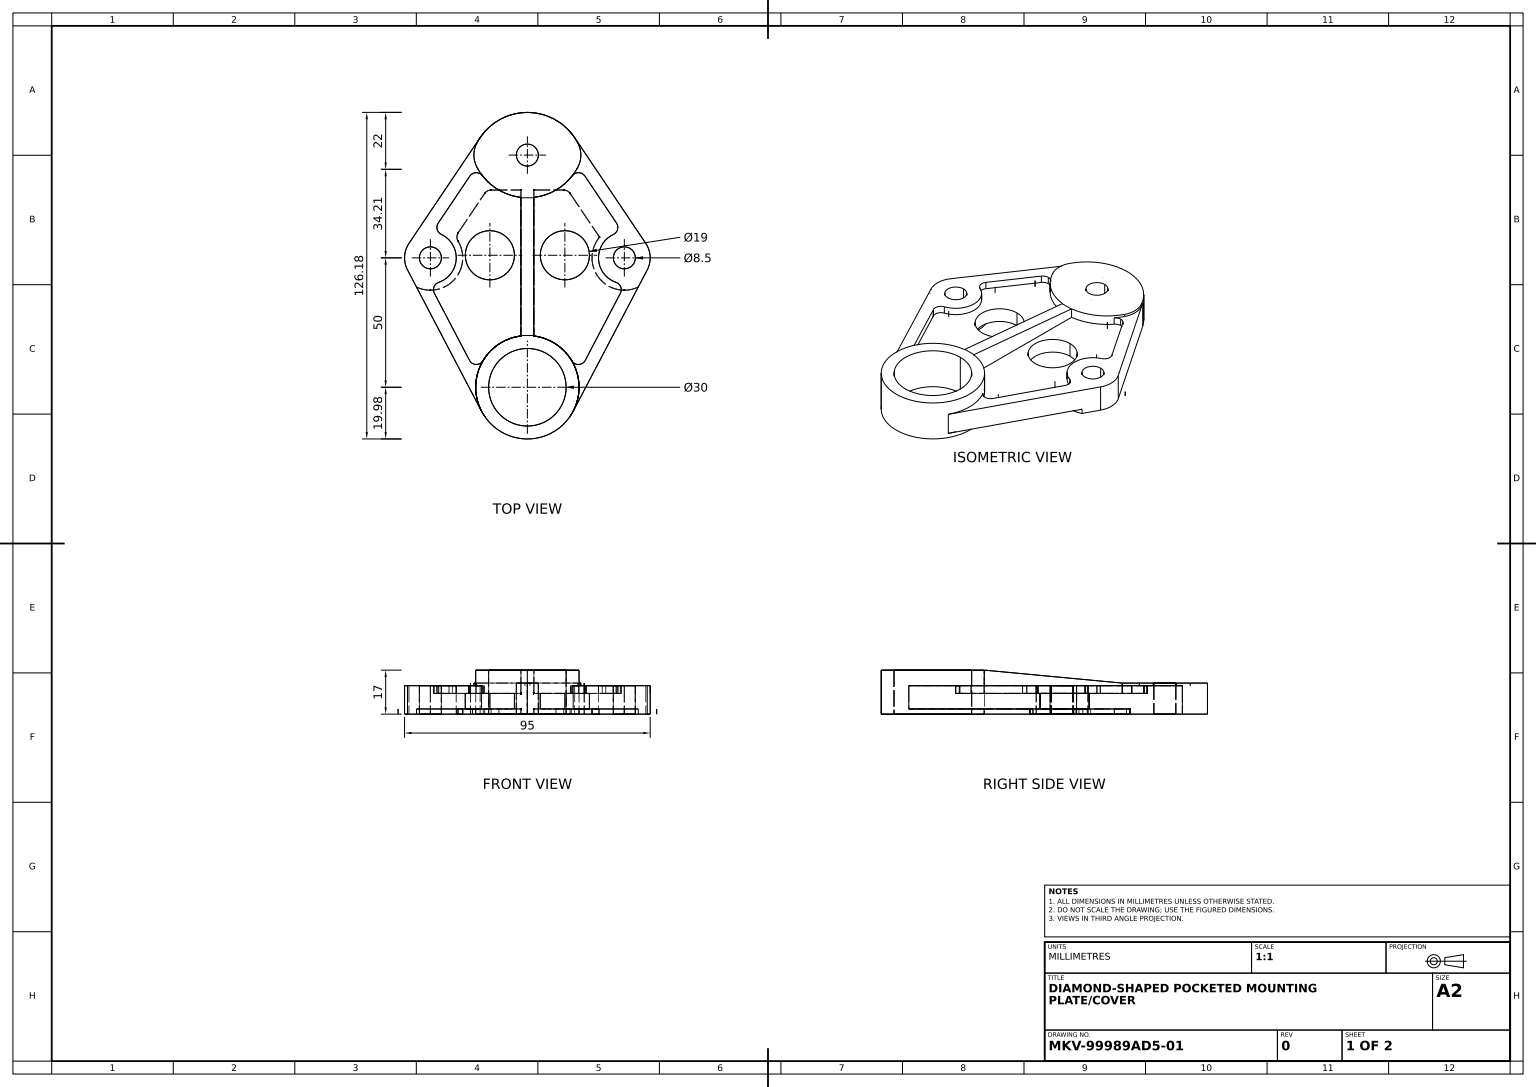
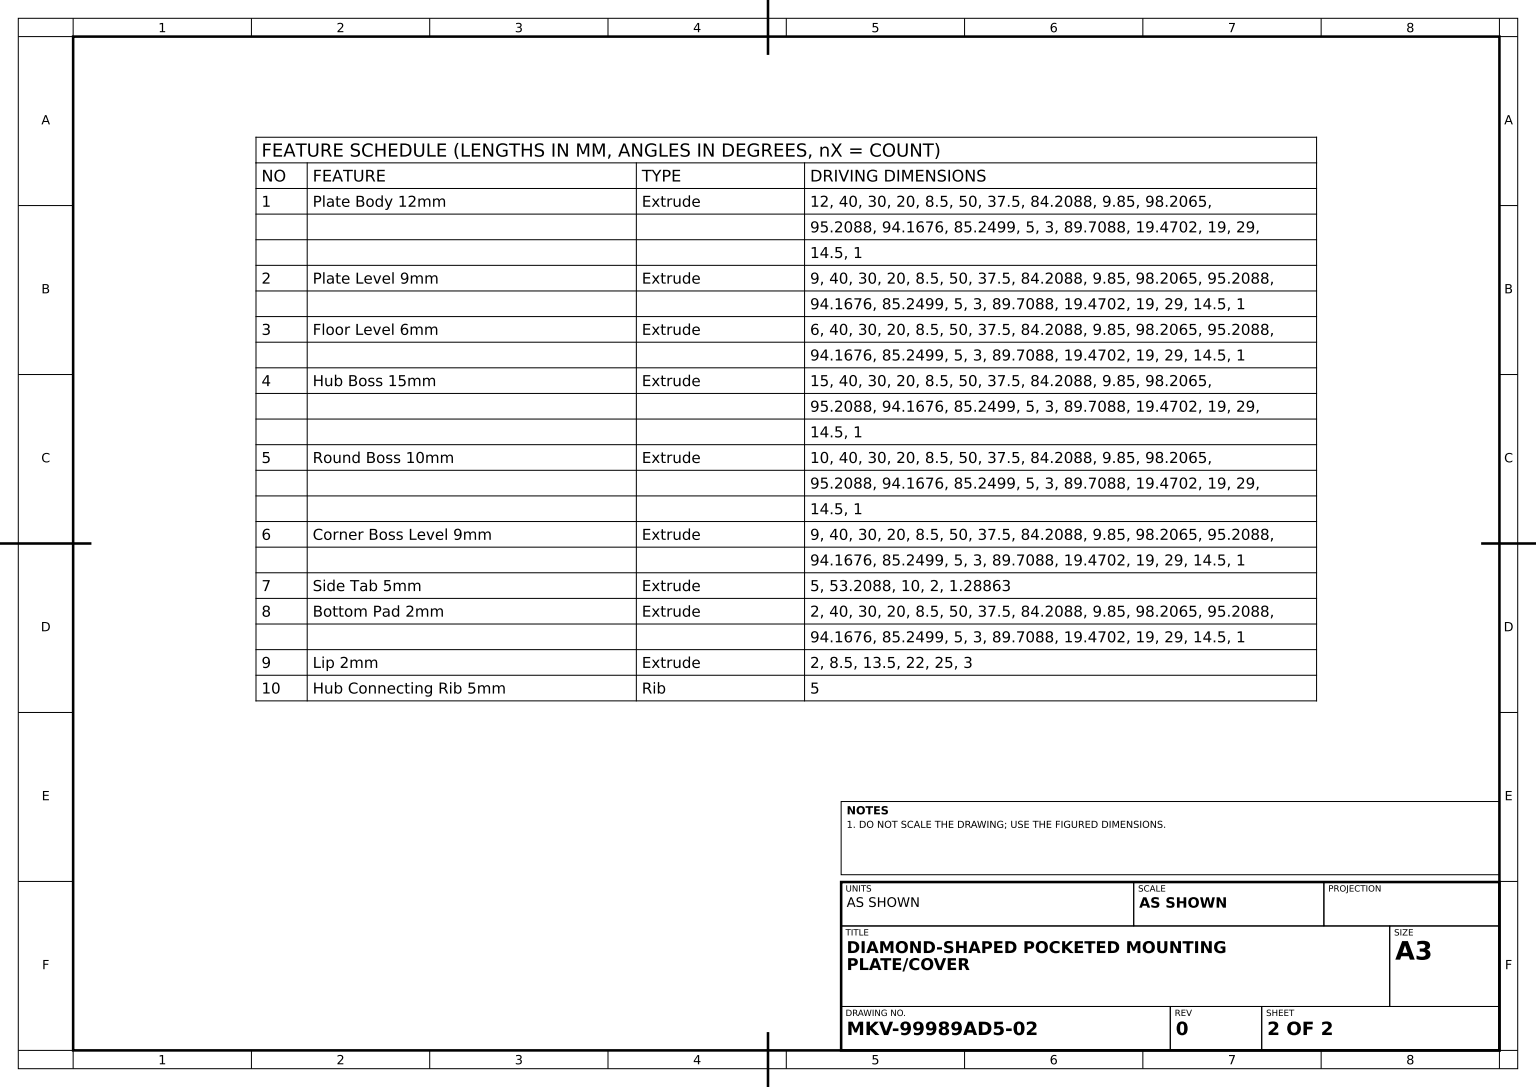
solid
v1 (-26.813948518,0,-56.485237369)
v2 (-37.5,0,-37.5)
e1 v1 v2 CIRCLE(AX(P(-37.5,0,-50),D(0,-1,0),D(0,0,-1)),12.5)
v3 (-37.5,-2,-37.5)
e2 v3 v2 LINE
v4 (-26.813948518,-2,-56.485237369)
e3 v4 v3 CIRCLE(AX(P(-37.5,-2,-50),D(0,-1,0),D(0,0,-1)),12.5)
e4 v4 v1 LINE
face CYL(AX(P(-37.5,-2,-50),D(0,1,0),D(0,0,1)),12.5) [e1 -e2 -e3 e4]
v5 (2.5,0,-19.843134833)
v6 (2.5,-2,-19.843134833)
e5 v5 v6 LINE
v7 (2.5,-2,-76.208782064)
e6 v7 v6 LINE
v8 (2.5,0,-76.208782064)
e7 v7 v8 LINE
e8 v8 v5 LINE
face PLANE(AX(P(2.5,-2,-20),D(-1,0,0),D(0,0,1))) rev [e5 -e6 e7 e8]
v9 (-14.5,0,-60.5)
v10 (-14.5,0,-41.5)
e9 v9 v10 CIRCLE(AX(P(-14.5,0,-51),D(0,1,0),D(0,0,1)),9.5)
e10 v10 v9 CIRCLE(AX(P(-14.5,0,-51),D(0,1,0),D(0,0,1)),9.5)
v11 (-26.737782046,0,-59.717235446)
e11 v1 v11 CIRCLE(AX(P(-24.249296162,0,-58.041694337),D(0,-1,0),D(0,0,-1)),3)
v12 (-16.525516364,0,-74.884323173)
e12 v11 v12 LINE
v13 (-14.037030481,0,-76.208782064)
e13 v13 v12 CIRCLE(AX(P(-14.037030481,0,-73.208782064),D(0,1,0),D(0,0,-1)),3)
v14 (-2.5,0,-76.208782064)
e14 v13 v14 LINE
v15 (-2.5,0,-19.843134833)
e15 v14 v15 LINE
v16 (-17.713872229,0,9.285404172)
e16 v15 v16 CIRCLE(AX(P(0,0,0),D(0,1,0),D(0,0,1)),20)
v17 (-42.87490955,0,-38.714595828)
e17 v17 v16 LINE
e18 v2 v17 CIRCLE(AX(P(-37.5,0,-50),D(0,-1,0),D(0,0,-1)),12.5)
face PLANE(AX(P(0,0,0),D(0,1,0),D(0,0,1))) rev [e9 e10] [-e1 e11 e12 -e13 e14 e15 e16 -e17 -e18]
v18 (-45.794952945,9,-55.58513703)
v19 (-46.356936115,9,-45.357297914)
e19 v18 v19 CIRCLE(AX(P(-37.5,9,-50),D(0,1,0),D(0,0,1)),10)
v20 (-45.794952945,-2,-55.58513703)
e20 v18 v20 LINE
v21 (-46.356936115,-2,-45.357297914)
e21 v21 v20 CIRCLE(AX(P(-37.5,-2,-50),D(0,-1,0),D(0,0,-1)),10)
e22 v19 v21 LINE
face CYL(AX(P(-37.5,6,-50),D(0,-1,0),D(0,0,-1)),10) [-e19 e20 -e21 -e22]
v22 (19.772275057,6,-82.909855988)
v23 (17.39960205,6,-81.745727117)
e23 v22 v23 CIRCLE(AX(P(19.772275057,6,-79.909855988),D(0,1,0),D(0,0,1)),3)
v24 (2.5,6,-73.351289069)
e24 v24 v23 CIRCLE(AX(P(0,6,-95.208782064),D(0,1,0),D(0,0,1)),22)
v25 (2.5,6,-19.843134833)
e25 v25 v24 LINE
v26 (17.163445775,6,-10.26723571)
e26 v26 v25 CIRCLE(AX(P(0,6,0),D(0,1,0),D(0,0,1)),20)
v27 (22.395043476,6,-10.414510441)
e27 v27 v26 CIRCLE(AX(P(19.737962641,6,-11.807321067),D(0,-1,0),D(0,0,1)),3)
v28 (35.964809248,6,-36.301708524)
e28 v28 v27 LINE
v29 (34.275175703,6,-40.5342455)
e29 v28 v29 CIRCLE(AX(P(33.307728414,6,-37.69451915),D(0,1,0),D(0,0,1)),3)
v30 (33.257501674,6,-59.055451836)
e30 v29 v30 CIRCLE(AX(P(37.5,6,-50),D(0,-1,0),D(0,0,1)),10)
v31 (34.47323806,6,-63.447628496)
e31 v30 v31 CIRCLE(AX(P(31.984752176,6,-61.772087387),D(0,1,0),D(0,0,1)),3)
v32 (22.26076094,6,-81.585397097)
e32 v31 v32 LINE
e33 v32 v22 CIRCLE(AX(P(19.772275057,6,-79.909855988),D(0,1,0),D(0,0,1)),3)
v33 (14.5,6,-60.5)
v34 (14.5,6,-41.5)
e34 v33 v34 CIRCLE(AX(P(14.5,6,-51),D(0,1,0),D(0,0,1)),9.5)
e35 v34 v33 CIRCLE(AX(P(14.5,6,-51),D(0,1,0),D(0,0,1)),9.5)
face PLANE(AX(P(0,6,0),D(0,1,0),D(0,0,1))) [e23 -e24 -e25 -e26 -e27 -e28 e29 e30 e31 e32 e33] [-e34 -e35]
v35 (-19.616863963,9,-94.1676298)
v36 (-19.616863963,9,-85.249934327)
e36 v35 v36 CIRCLE(AX(P(-10.833858962,9,-89.708782064),D(0,1,0),D(0,0,1)),9.85)
v37 (-19.616863963,10,-85.249934327)
e37 v37 v36 LINE
v38 (-19.616863963,10,-94.1676298)
e38 v38 v37 CIRCLE(AX(P(-10.833858962,10,-89.708782064),D(0,1,0),D(0,0,1)),9.85)
e39 v38 v35 LINE
face CYL(AX(P(-10.833858962,9,-89.708782064),D(0,-1,0),D(0,0,-1)),9.85) [e36 -e37 -e38 e39]
v39 (0,15,15)
v40 (0,15,-15)
e40 v39 v40 CIRCLE(AX(P(0,15,0),D(0,1,0),D(0,0,1)),15)
e41 v40 v39 CIRCLE(AX(P(0,15,0),D(0,1,0),D(0,0,1)),15)
v41 (-2.5,15,-19.843134833)
v42 (2.5,15,-19.843134833)
e42 v41 v42 CIRCLE(AX(P(0,15,0),D(0,1,0),D(0,0,1)),20)
v43 (2.5,15,-20)
e43 v43 v42 LINE
v44 (-2.5,15,-20)
e44 v43 v44 LINE
e45 v44 v41 LINE
face PLANE(AX(P(0,15,0),D(0,1,0),D(0,0,1))) [-e40 -e41] [e42 -e43 e44 e45]
v45 (16.525516364,0,-74.884323173)
v46 (27.894602034,0,-57.999145574)
e46 v45 v46 LINE
v47 (16.525516364,-2,-74.884323173)
e47 v47 v45 LINE
v48 (27.894602034,-2,-57.999145574)
e48 v47 v48 LINE
e49 v48 v46 LINE
face PLANE(AX(P(46.063332531,-2,-31.015248179),D(-0.829495295,0,0.558513703),D(0.558513703,0,0.829495295))) [-e46 -e47 e48 e49]
v49 (-2.5,6,-19.843134833)
e50 v49 v41 LINE
v50 (-2.5,10,-73.208782064)
e51 v50 v44 LINE
v51 (-2.5,10,-73.351289069)
e52 v51 v50 LINE
v52 (-2.5,6,-73.351289069)
e53 v51 v52 LINE
e54 v49 v52 LINE
face PLANE(AX(P(-2.5,0,0),D(1,0,0),D(0,0,-1))) rev [e50 -e45 -e51 -e52 e53 -e54]
v53 (-17.713872229,9,9.285404172)
e55 v53 v16 LINE
e56 v19 v53 LINE
v54 (-42.87490955,-2,-38.714595828)
e57 v54 v21 LINE
e58 v54 v17 LINE
face PLANE(AX(P(-17.713872229,6,9.285404172),D(0.885693611,0,-0.464270209),D(-0.464270209,0,-0.885693611))) rev [-e55 -e56 e22 -e57 e58 e17]
v55 (34.275175703,9,-40.5342455)
v56 (35.964809248,9,-36.301708524)
e59 v55 v56 CIRCLE(AX(P(33.307728414,9,-37.69451915),D(0,-1,0),D(0,0,1)),3)
e60 v55 v29 LINE
e61 v56 v28 LINE
face CYL(AX(P(33.307728414,9,-37.69451915),D(0,-1,0),D(0,0,-1)),3) rev [-e59 e60 -e29 -e61]
v57 (-18.248896479,9,-96.496083529)
e62 v18 v57 LINE
v58 (-17.163445775,9,-10.26723571)
e63 v58 v53 CIRCLE(AX(P(0,9,0),D(0,1,0),D(0,0,1)),20)
v59 (-22.395043476,9,-10.414510441)
e64 v59 v58 CIRCLE(AX(P(-19.737962641,9,-11.807321067),D(0,1,0),D(0,0,1)),3)
v60 (-35.964809248,9,-36.301708524)
e65 v60 v59 LINE
v61 (-34.275175703,9,-40.5342455)
e66 v61 v60 CIRCLE(AX(P(-33.307728414,9,-37.69451915),D(0,1,0),D(0,0,1)),3)
v62 (-33.257501674,9,-59.055451836)
e67 v61 v62 CIRCLE(AX(P(-37.5,9,-50),D(0,1,0),D(0,0,1)),10)
v63 (-34.47323806,9,-63.447628496)
e68 v63 v62 CIRCLE(AX(P(-31.984752176,9,-61.772087387),D(0,1,0),D(0,0,1)),3)
v64 (-22.26076094,9,-81.585397097)
e69 v63 v64 LINE
v65 (-19.772275057,9,-82.909855988)
e70 v64 v65 CIRCLE(AX(P(-19.772275057,9,-79.909855988),D(0,-1,0),D(0,0,1)),3)
v66 (-17.39960205,9,-81.745727117)
e71 v65 v66 CIRCLE(AX(P(-19.772275057,9,-79.909855988),D(0,-1,0),D(0,0,1)),3)
e72 v36 v66 CIRCLE(AX(P(0,9,-95.208782064),D(0,1,0),D(0,0,1)),22)
e73 v57 v35 CIRCLE(AX(P(0,9,-84.208782064),D(0,1,0),D(0,0,1)),22)
v67 (-37.5,9,-54.25)
v68 (-37.5,9,-45.75)
e74 v67 v68 CIRCLE(AX(P(-37.5,9,-50),D(0,1,0),D(0,0,1)),4.25)
e75 v68 v67 CIRCLE(AX(P(-37.5,9,-50),D(0,1,0),D(0,0,1)),4.25)
face PLANE(AX(P(0,9,0),D(0,1,0),D(0,0,1))) [-e62 e19 e56 -e63 -e64 -e65 -e66 e67 -e68 e69 e70 e71 -e72 -e36 -e73] [-e74 -e75]
v69 (-18.248896479,-2,-96.496083529)
e76 v20 v69 LINE
e77 v57 v69 LINE
face PLANE(AX(P(-57.261519006,6,-38.555183168),D(-0.829495295,0,-0.558513703),D(-0.558513703,0,0.829495295))) [-e76 -e20 e62 e77]
v70 (19.616863963,9,-94.1676298)
v71 (19.616863963,9,-85.249934327)
e78 v70 v71 CIRCLE(AX(P(10.833858962,9,-89.708782064),D(0,-1,0),D(0,0,1)),9.85)
v72 (19.616863963,10,-94.1676298)
e79 v72 v70 LINE
v73 (19.616863963,10,-85.249934327)
e80 v72 v73 CIRCLE(AX(P(10.833858962,10,-89.708782064),D(0,-1,0),D(0,0,1)),9.85)
e81 v73 v71 LINE
face CYL(AX(P(10.833858962,9,-89.708782064),D(0,-1,0),D(0,0,-1)),9.85) [-e78 -e79 e80 e81]
v74 (-22.395043476,6,-10.414510441)
e82 v59 v74 LINE
v75 (-35.964809248,6,-36.301708524)
e83 v74 v75 LINE
e84 v60 v75 LINE
face PLANE(AX(P(-13.285404172,9,6.964053129),D(0.885693611,0,-0.464270209),D(-0.464270209,0,-0.885693611))) [e82 e83 -e84 e65]
v76 (33.257501674,9,-59.055451836)
e85 v76 v55 CIRCLE(AX(P(37.5,9,-50),D(0,1,0),D(0,0,1)),10)
e86 v76 v30 LINE
face CYL(AX(P(37.5,9,-50),D(0,-1,0),D(0,0,-1)),10) [-e60 -e85 e86 -e30]
v77 (0,-2,15)
e87 v39 v77 LINE
v78 (0,-2,-15)
e88 v78 v77 CIRCLE(AX(P(0,-2,0),D(0,1,0),D(0,0,1)),15)
e89 v40 v78 LINE
face CYL(AX(P(0,12,0),D(0,-1,0),D(0,0,-1)),15) rev [e87 -e88 -e89 e41]
v79 (0,10,-106.208782064)
e90 v79 v38 CIRCLE(AX(P(0,10,-84.208782064),D(0,1,0),D(0,0,1)),22)
v80 (0,-2,-106.208782064)
e91 v79 v80 LINE
e92 v69 v80 CIRCLE(AX(P(0,-2,-84.208782064),D(0,-1,0),D(0,0,-1)),22)
face CYL(AX(P(0,9,-84.208782064),D(0,-1,0),D(0,0,-1)),22) [e73 -e39 -e90 e91 -e92 -e77]
v81 (46.356936115,9,-45.357297914)
v82 (46.356936115,-2,-45.357297914)
e93 v81 v82 LINE
v83 (45.794952945,-2,-55.58513703)
e94 v83 v82 CIRCLE(AX(P(37.5,-2,-50),D(0,-1,0),D(0,0,-1)),10)
v84 (45.794952945,9,-55.58513703)
e95 v84 v83 LINE
e96 v81 v84 CIRCLE(AX(P(37.5,9,-50),D(0,1,0),D(0,0,1)),10)
face CYL(AX(P(37.5,6,-50),D(0,-1,0),D(0,0,-1)),10) [e93 -e94 -e95 -e96]
v85 (34.47323806,9,-63.447628496)
e97 v85 v76 CIRCLE(AX(P(31.984752176,9,-61.772087387),D(0,-1,0),D(0,0,1)),3)
e98 v85 v31 LINE
face CYL(AX(P(31.984752176,9,-61.772087387),D(0,-1,0),D(0,0,-1)),3) rev [-e86 -e97 e98 -e31]
v86 (0,10,-93.958782064)
v87 (0,10,-85.458782064)
e99 v86 v87 CIRCLE(AX(P(0,10,-89.708782064),D(0,1,0),D(0,0,1)),4.25)
v88 (0,-2,-85.458782064)
e100 v87 v88 LINE
v89 (0,-2,-93.958782064)
e101 v89 v88 CIRCLE(AX(P(0,-2,-89.708782064),D(0,1,0),D(0,0,-1)),4.25)
e102 v86 v89 LINE
face CYL(AX(P(0,9,-89.708782064),D(0,-1,0),D(0,0,-1)),4.25) rev [e99 e100 -e101 -e102]
v90 (17.39960205,9,-81.745727117)
v91 (19.772275057,9,-82.909855988)
e103 v90 v91 CIRCLE(AX(P(19.772275057,9,-79.909855988),D(0,-1,0),D(0,0,1)),3)
e104 v90 v23 LINE
e105 v91 v22 LINE
face CYL(AX(P(19.772275057,9,-79.909855988),D(0,-1,0),D(0,0,-1)),3) rev [-e103 e104 -e23 -e105]
v92 (22.26076094,9,-81.585397097)
e106 v92 v85 LINE
e107 v92 v32 LINE
face PLANE(AX(P(53.114042534,9,-35.762614654),D(0.829495295,0,-0.558513703),D(-0.558513703,0,-0.829495295))) rev [-e106 e107 -e32 -e98]
v93 (37.5,9,-54.25)
v94 (37.5,-2,-54.25)
e108 v93 v94 LINE
v95 (37.5,9,-45.75)
e109 v93 v95 CIRCLE(AX(P(37.5,9,-50),D(0,1,0),D(0,0,1)),4.25)
v96 (37.5,-2,-45.75)
e110 v95 v96 LINE
e111 v94 v96 CIRCLE(AX(P(37.5,-2,-50),D(0,1,0),D(0,0,-1)),4.25)
face CYL(AX(P(37.5,6,-50),D(0,-1,0),D(0,0,-1)),4.25) rev [-e108 e109 e110 -e111]
v97 (-33.257501674,6,-59.055451836)
e112 v62 v97 LINE
v98 (-34.47323806,6,-63.447628496)
e113 v97 v98 CIRCLE(AX(P(-31.984752176,6,-61.772087387),D(0,-1,0),D(0,0,1)),3)
e114 v63 v98 LINE
face CYL(AX(P(-31.984752176,9,-61.772087387),D(0,-1,0),D(0,0,-1)),3) rev [e112 e113 -e114 e68]
v99 (2.5,10,-73.208782064)
e115 v99 v43 LINE
e116 v25 v42 LINE
v100 (2.5,10,-73.351289069)
e117 v100 v24 LINE
e118 v100 v99 LINE
face PLANE(AX(P(2.5,0,0),D(1,0,0),D(0,0,-1))) [e115 e43 -e116 e25 -e117 e118]
v101 (-26.737782046,-2,-59.717235446)
v102 (-16.525516364,-2,-74.884323173)
e119 v101 v102 LINE
e120 v102 v12 LINE
e121 v101 v11 LINE
face PLANE(AX(P(-46.063332531,-2,-31.015248179),D(0.829495295,0,0.558513703),D(0.558513703,0,-0.829495295))) [e119 e120 -e12 -e121]
v103 (-22.26076094,6,-81.585397097)
e122 v64 v103 LINE
v104 (-19.772275057,6,-82.909855988)
e123 v104 v103 CIRCLE(AX(P(-19.772275057,6,-79.909855988),D(0,1,0),D(0,0,1)),3)
e124 v65 v104 LINE
face CYL(AX(P(-19.772275057,9,-79.909855988),D(0,-1,0),D(0,0,-1)),3) rev [e122 -e123 -e124 -e70]
v105 (-34.275175703,6,-40.5342455)
e125 v61 v105 LINE
e126 v75 v105 CIRCLE(AX(P(-33.307728414,6,-37.69451915),D(0,-1,0),D(0,0,1)),3)
face CYL(AX(P(-33.307728414,9,-37.69451915),D(0,-1,0),D(0,0,-1)),3) rev [-e125 e66 e84 e126]
v106 (-37.5,-2,-45.75)
e127 v68 v106 LINE
v107 (-37.5,-2,-54.25)
e128 v67 v107 LINE
e129 v106 v107 CIRCLE(AX(P(-37.5,-2,-50),D(0,1,0),D(0,0,-1)),4.25)
face CYL(AX(P(-37.5,6,-50),D(0,-1,0),D(0,0,-1)),4.25) rev [-e127 e75 e128 -e129]
v108 (-2.5,-2,-76.208782064)
v109 (-2.5,-2,-19.843134833)
e130 v108 v109 LINE
e131 v15 v109 LINE
e132 v108 v14 LINE
face PLANE(AX(P(-2.5,-2,-20),D(-1,0,0),D(0,0,1))) [e130 -e131 -e15 -e132]
v110 (-14.037030481,-2,-76.208782064)
e133 v110 v108 LINE
e134 v110 v13 LINE
face PLANE(AX(P(0,-2,-76.208782064),D(0,0,1),D(1,0,0))) [e133 e132 -e14 -e134]
e135 v3 v54 CIRCLE(AX(P(-37.5,-2,-50),D(0,-1,0),D(0,0,-1)),12.5)
face CYL(AX(P(-37.5,-2,-50),D(0,1,0),D(0,0,1)),12.5) [e2 e18 -e58 -e135]
e136 v107 v106 CIRCLE(AX(P(-37.5,-2,-50),D(0,1,0),D(0,0,-1)),4.25)
face CYL(AX(P(-37.5,6,-50),D(0,-1,0),D(0,0,-1)),4.25) rev [e127 -e136 -e128 e74]
v111 (14.5,0,-41.5)
e137 v34 v111 LINE
v112 (14.5,0,-60.5)
e138 v112 v111 CIRCLE(AX(P(14.5,0,-51),D(0,1,0),D(0,0,1)),9.5)
e139 v33 v112 LINE
face CYL(AX(P(14.5,6,-51),D(0,-1,0),D(0,0,-1)),9.5) rev [e137 -e138 -e139 e34]
e140 v4 v101 CIRCLE(AX(P(-24.249296162,-2,-58.041694337),D(0,-1,0),D(0,0,-1)),3)
face CYL(AX(P(-24.249296162,-2,-58.041694337),D(0,1,0),D(0,0,1)),3) rev [-e11 -e4 e140 e121]
v113 (17.163445775,9,-10.26723571)
e141 v113 v26 LINE
v114 (22.395043476,9,-10.414510441)
e142 v113 v114 CIRCLE(AX(P(19.737962641,9,-11.807321067),D(0,1,0),D(0,0,1)),3)
e143 v114 v27 LINE
face CYL(AX(P(19.737962641,9,-11.807321067),D(0,-1,0),D(0,0,-1)),3) rev [-e141 e142 e143 e27]
e144 v103 v98 LINE
face PLANE(AX(P(-53.114042534,9,-35.762614654),D(-0.829495295,0,-0.558513703),D(-0.558513703,0,0.829495295))) rev [e114 -e144 -e122 -e69]
e145 v72 v79 CIRCLE(AX(P(0,10,-84.208782064),D(0,1,0),D(0,0,1)),22)
v115 (18.248896479,9,-96.496083529)
e146 v70 v115 CIRCLE(AX(P(0,9,-84.208782064),D(0,1,0),D(0,0,1)),22)
v116 (18.248896479,-2,-96.496083529)
e147 v115 v116 LINE
e148 v80 v116 CIRCLE(AX(P(0,-2,-84.208782064),D(0,-1,0),D(0,0,-1)),22)
face CYL(AX(P(0,9,-84.208782064),D(0,-1,0),D(0,0,-1)),22) [-e91 -e145 e79 e146 e147 -e148]
e149 v97 v105 CIRCLE(AX(P(-37.5,6,-50),D(0,-1,0),D(0,0,1)),10)
face CYL(AX(P(-37.5,9,-50),D(0,-1,0),D(0,0,-1)),10) [-e67 e125 -e149 -e112]
e150 v109 v6 CIRCLE(AX(P(0,-2,0),D(0,1,0),D(0,0,1)),20)
v117 (17.713872229,0,9.285404172)
e151 v117 v5 CIRCLE(AX(P(0,0,0),D(0,1,0),D(0,0,1)),20)
v118 (17.713872229,9,9.285404172)
e152 v118 v117 LINE
e153 v118 v113 CIRCLE(AX(P(0,9,0),D(0,1,0),D(0,0,1)),20)
v119 (-17.163445775,6,-10.26723571)
e154 v49 v119 CIRCLE(AX(P(0,6,0),D(0,1,0),D(0,0,1)),20)
e155 v58 v119 LINE
face CYL(AX(P(0,12,0),D(0,-1,0),D(0,0,-1)),20) [e63 e55 -e16 e131 e150 -e5 -e151 -e152 e153 e141 e26 e116 -e42 -e50 e154 -e155]
e156 v95 v93 CIRCLE(AX(P(37.5,9,-50),D(0,1,0),D(0,0,1)),4.25)
e157 v118 v81 LINE
e158 v115 v84 LINE
e159 v90 v71 CIRCLE(AX(P(0,9,-95.208782064),D(0,1,0),D(0,0,1)),22)
e160 v91 v92 CIRCLE(AX(P(19.772275057,9,-79.909855988),D(0,-1,0),D(0,0,1)),3)
e161 v114 v56 LINE
face PLANE(AX(P(0,9,0),D(0,1,0),D(0,0,1))) [-e109 -e156] [-e153 e157 e96 -e158 -e146 e78 -e159 e103 e160 e106 e97 e85 e59 -e161 -e142]
e162 v116 v83 LINE
v120 (42.87490955,-2,-38.714595828)
e163 v82 v120 LINE
v121 (37.5,-2,-37.5)
e164 v120 v121 CIRCLE(AX(P(37.5,-2,-50),D(0,-1,0),D(0,0,-1)),12.5)
e165 v121 v48 CIRCLE(AX(P(37.5,-2,-50),D(0,-1,0),D(0,0,-1)),12.5)
v122 (14.037030481,-2,-76.208782064)
e166 v47 v122 CIRCLE(AX(P(14.037030481,-2,-73.208782064),D(0,1,0),D(0,0,-1)),3)
e167 v7 v122 LINE
e168 v110 v102 CIRCLE(AX(P(-14.037030481,-2,-73.208782064),D(0,1,0),D(0,0,-1)),3)
e169 v88 v89 CIRCLE(AX(P(0,-2,-89.708782064),D(0,1,0),D(0,0,-1)),4.25)
e170 v77 v78 CIRCLE(AX(P(0,-2,0),D(0,1,0),D(0,0,1)),15)
e171 v96 v94 CIRCLE(AX(P(37.5,-2,-50),D(0,1,0),D(0,0,-1)),4.25)
face PLANE(AX(P(0,-2,0),D(0,1,0),D(0,0,1))) rev [e135 e57 e21 e76 e92 e148 e162 e94 e163 e164 e165 -e48 e166 -e167 e6 -e150 -e130 -e133 e168 -e119 -e140 e3] [e101 e169] [e88 e170] [e136 e129] [e111 e171]
e172 v99 v50 LINE
face PLANE(AX(P(2.5,15,-20),D(0,-0.995613898,0.093557291),D(0,-0.093557291,-0.995613898))) rev [e172 e51 -e44 -e115]
face CYL(AX(P(19.772275057,9,-79.909855988),D(0,-1,0),D(0,0,-1)),3) rev [e105 -e33 -e107 -e160]
e173 v37 v51 CIRCLE(AX(P(0,10,-95.208782064),D(0,1,0),D(0,0,1)),22)
v123 (-17.39960205,6,-81.745727117)
e174 v66 v123 LINE
e175 v123 v52 CIRCLE(AX(P(0,6,-95.208782064),D(0,1,0),D(0,0,1)),22)
face CYL(AX(P(0,9,-95.208782064),D(0,-1,0),D(0,0,-1)),22) [-e53 -e173 e37 e72 e174 e175]
e176 v100 v73 CIRCLE(AX(P(0,10,-95.208782064),D(0,1,0),D(0,0,1)),22)
face CYL(AX(P(0,9,-95.208782064),D(0,-1,0),D(0,0,-1)),22) [e117 e24 -e104 e159 -e81 -e176]
face CYL(AX(P(-14.037030481,-2,-73.208782064),D(0,1,0),D(0,0,1)),3) rev [-e120 -e168 e134 e13]
v124 (14.037030481,0,-76.208782064)
e177 v45 v124 CIRCLE(AX(P(14.037030481,0,-73.208782064),D(0,1,0),D(0,0,-1)),3)
e178 v122 v124 LINE
face CYL(AX(P(14.037030481,-2,-73.208782064),D(0,1,0),D(0,0,1)),3) rev [-e166 e47 e177 -e178]
face CYL(AX(P(37.5,6,-50),D(0,-1,0),D(0,0,-1)),4.25) rev [-e110 e156 e108 -e171]
e179 v119 v74 CIRCLE(AX(P(-19.737962641,6,-11.807321067),D(0,-1,0),D(0,0,1)),3)
face CYL(AX(P(-19.737962641,9,-11.807321067),D(0,-1,0),D(0,0,-1)),3) rev [e155 e179 -e82 e64]
e180 v123 v104 CIRCLE(AX(P(-19.772275057,6,-79.909855988),D(0,1,0),D(0,0,1)),3)
face CYL(AX(P(-19.772275057,9,-79.909855988),D(0,-1,0),D(0,0,-1)),3) rev [-e71 e124 -e180 -e174]
v125 (37.5,0,-37.5)
e181 v125 v46 CIRCLE(AX(P(37.5,0,-50),D(0,-1,0),D(0,0,-1)),12.5)
v126 (42.87490955,0,-38.714595828)
e182 v126 v125 CIRCLE(AX(P(37.5,0,-50),D(0,-1,0),D(0,0,-1)),12.5)
e183 v117 v126 LINE
e184 v8 v124 LINE
e185 v111 v112 CIRCLE(AX(P(14.5,0,-51),D(0,1,0),D(0,0,1)),9.5)
face PLANE(AX(P(0,0,0),D(0,1,0),D(0,0,1))) rev [-e181 -e182 -e183 e151 -e8 e184 -e177 e46] [e185 e138]
v127 (-14.5,6,-60.5)
v128 (-14.5,6,-41.5)
e186 v127 v128 CIRCLE(AX(P(-14.5,6,-51),D(0,1,0),D(0,0,1)),9.5)
e187 v128 v127 CIRCLE(AX(P(-14.5,6,-51),D(0,1,0),D(0,0,1)),9.5)
face PLANE(AX(P(0,6,0),D(0,1,0),D(0,0,1))) [-e154 e54 -e175 e180 e123 e144 -e113 e149 -e126 -e83 -e179] [-e186 -e187]
face CYL(AX(P(14.5,6,-51),D(0,-1,0),D(0,0,-1)),9.5) rev [e139 -e185 -e137 e35]
face CYL(AX(P(0,12,0),D(0,-1,0),D(0,0,-1)),15) rev [-e170 -e87 e40 e89]
e188 v87 v86 CIRCLE(AX(P(0,10,-89.708782064),D(0,1,0),D(0,0,1)),4.25)
face PLANE(AX(P(0,10,0),D(0,1,0),D(0,0,1))) [-e99 -e188] [-e172 -e118 e176 -e80 e145 e90 e38 e173 e52]
face PLANE(AX(P(57.261519006,6,-38.555183168),D(0.829495295,0,-0.558513703),D(-0.558513703,0,-0.829495295))) [-e147 e158 e95 -e162]
e189 v121 v125 LINE
face CYL(AX(P(37.5,-2,-50),D(0,1,0),D(0,0,1)),12.5) [-e49 -e165 e189 e181]
face PLANE(AX(P(13.285404172,9,6.964053129),D(-0.885693611,0,-0.464270209),D(-0.464270209,0,0.885693611))) [e161 e61 e28 -e143]
e190 v127 v9 LINE
e191 v128 v10 LINE
face CYL(AX(P(-14.5,6,-51),D(0,-1,0),D(0,0,-1)),9.5) rev [e190 -e10 -e191 e187]
e192 v120 v126 LINE
face CYL(AX(P(37.5,-2,-50),D(0,1,0),D(0,0,1)),12.5) [e192 e182 -e189 -e164]
face PLANE(AX(P(0,-2,-76.208782064),D(0,0,1),D(1,0,0))) [-e184 -e7 e167 e178]
face PLANE(AX(P(17.713872229,6,9.285404172),D(-0.885693611,0,-0.464270209),D(-0.464270209,0,0.885693611))) rev [-e93 -e157 e152 e183 -e192 -e163]
face CYL(AX(P(0,9,-89.708782064),D(0,-1,0),D(0,0,-1)),4.25) rev [e188 e102 -e169 -e100]
face CYL(AX(P(-14.5,6,-51),D(0,-1,0),D(0,0,-1)),9.5) rev [-e9 -e190 e186 e191]
